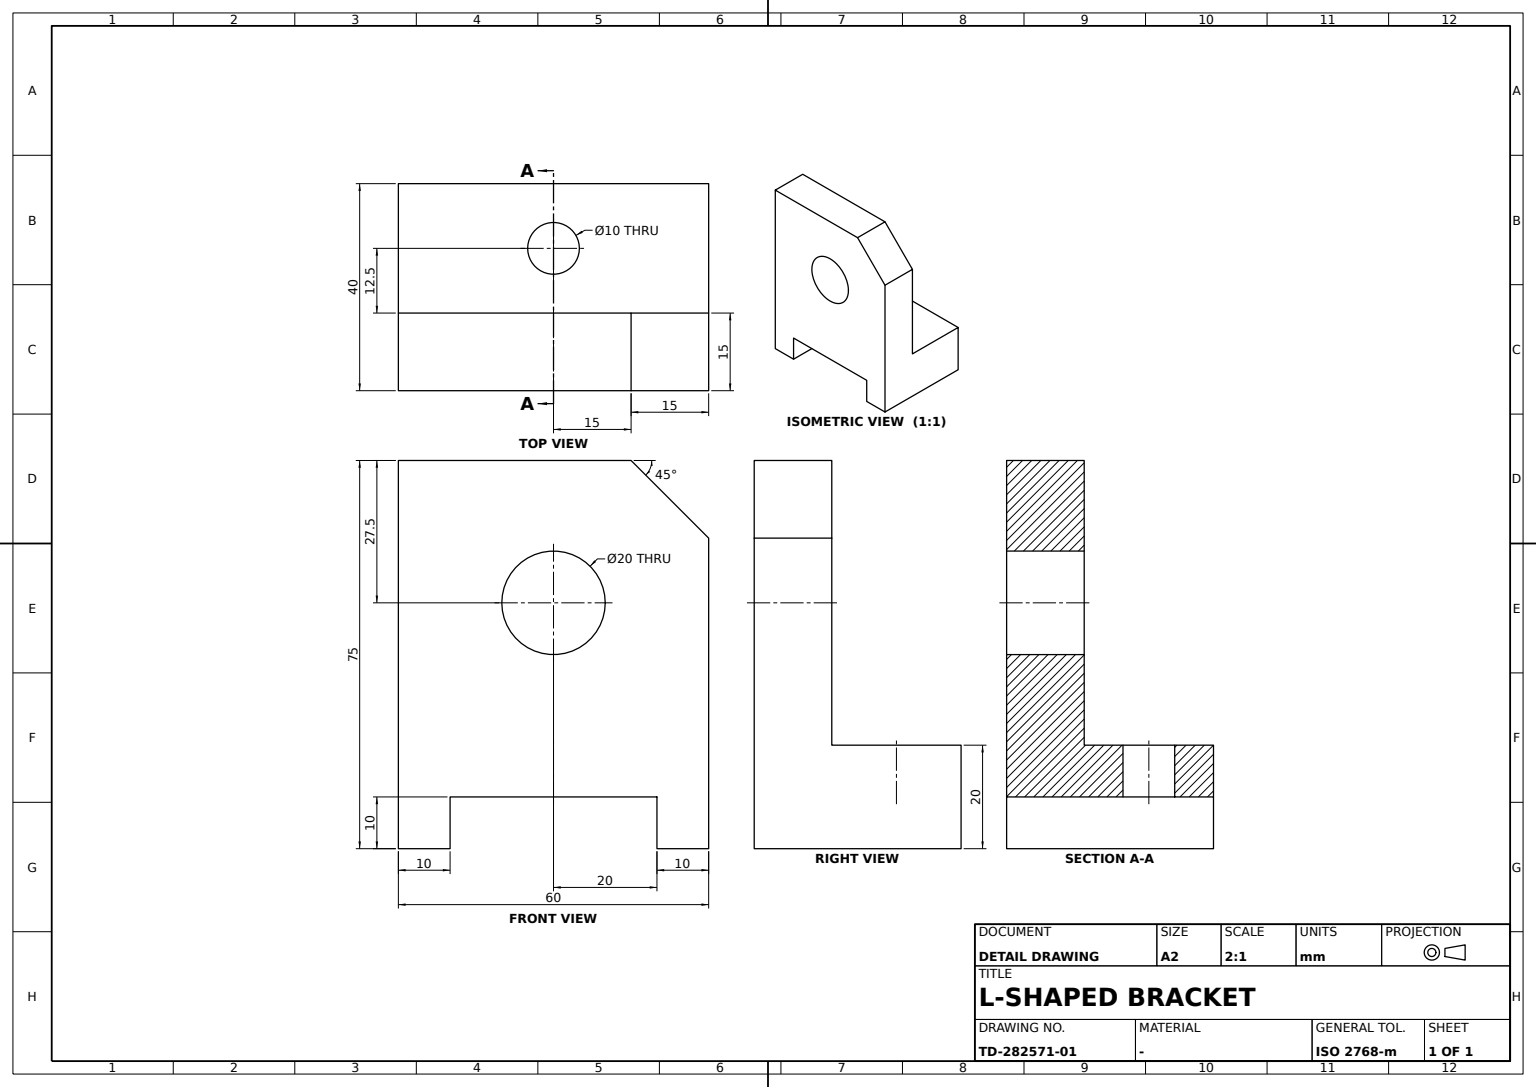
ISO-10303-21;
HEADER;
FILE_DESCRIPTION((''),'2;1');
FILE_NAME('','',(''),(''),'','','');
FILE_SCHEMA(('AUTOMOTIVE_DESIGN'));
ENDSEC;
DATA;
#1=APPLICATION_CONTEXT('');
#2=PRODUCT_CONTEXT('',#1,'mechanical');
#3=PRODUCT('','','',(#2));
#4=PRODUCT_DEFINITION_FORMATION('','',#3);
#5=PRODUCT_DEFINITION_CONTEXT('',#1,'design');
#6=PRODUCT_DEFINITION('','',#4,#5);
#7=PRODUCT_DEFINITION_SHAPE('','',#6);
#8=(LENGTH_UNIT()NAMED_UNIT(*)SI_UNIT(.MILLI.,.METRE.));
#9=(NAMED_UNIT(*)PLANE_ANGLE_UNIT()SI_UNIT($,.RADIAN.));
#10=(NAMED_UNIT(*)SI_UNIT($,.STERADIAN.)SOLID_ANGLE_UNIT());
#11=UNCERTAINTY_MEASURE_WITH_UNIT(LENGTH_MEASURE(1.E-05),#8,'distance_accuracy_value','');
#12=(GEOMETRIC_REPRESENTATION_CONTEXT(3)GLOBAL_UNCERTAINTY_ASSIGNED_CONTEXT((#11))GLOBAL_UNIT_ASSIGNED_CONTEXT((#8,#9,#10))REPRESENTATION_CONTEXT('',''));
#13=CARTESIAN_POINT('',(-20.,20.,10.));
#14=VERTEX_POINT('',#13);
#15=CARTESIAN_POINT('',(20.,20.,10.));
#16=VERTEX_POINT('',#15);
#17=CARTESIAN_POINT('',(0.,20.,10.));
#18=DIRECTION('',(1.,0.,0.));
#19=VECTOR('',#18,1000.);
#20=LINE('',#17,#19);
#21=EDGE_CURVE('',#14,#16,#20,.T.);
#22=ORIENTED_EDGE('',*,*,#21,.T.);
#23=CARTESIAN_POINT('',(20.,-20.,10.));
#24=VERTEX_POINT('',#23);
#25=CARTESIAN_POINT('',(20.,0.,10.));
#26=DIRECTION('',(0.,-1.,0.));
#27=VECTOR('',#26,1000.);
#28=LINE('',#25,#27);
#29=EDGE_CURVE('',#16,#24,#28,.T.);
#30=ORIENTED_EDGE('',*,*,#29,.T.);
#31=CARTESIAN_POINT('',(-20.,-20.,10.));
#32=VERTEX_POINT('',#31);
#33=CARTESIAN_POINT('',(0.,-20.,10.));
#34=DIRECTION('',(-1.,0.,0.));
#35=VECTOR('',#34,1000.);
#36=LINE('',#33,#35);
#37=EDGE_CURVE('',#24,#32,#36,.T.);
#38=ORIENTED_EDGE('',*,*,#37,.T.);
#39=CARTESIAN_POINT('',(-20.,0.,10.));
#40=LINE('',#39,#27);
#41=EDGE_CURVE('',#14,#32,#40,.T.);
#42=ORIENTED_EDGE('',*,*,#41,.F.);
#43=EDGE_LOOP('',(#22,#30,#38,#42));
#44=FACE_OUTER_BOUND('',#43,.T.);
#45=CARTESIAN_POINT('',(-5.,7.5,10.));
#46=VERTEX_POINT('',#45);
#47=CARTESIAN_POINT('',(5.,7.5,10.));
#48=VERTEX_POINT('',#47);
#49=CARTESIAN_POINT('',(0.,7.5,10.));
#50=DIRECTION('',(0.,0.,1.));
#51=AXIS2_PLACEMENT_3D('',#49,#50,#34);
#52=CIRCLE('',#51,5.);
#53=EDGE_CURVE('',#46,#48,#52,.T.);
#54=ORIENTED_EDGE('',*,*,#53,.T.);
#55=EDGE_CURVE('',#48,#46,#52,.T.);
#56=ORIENTED_EDGE('',*,*,#55,.T.);
#57=EDGE_LOOP('',(#54,#56));
#58=FACE_BOUND('',#57,.T.);
#59=AXIS2_PLACEMENT_3D('',#15,#50,#34);
#60=PLANE('',#59);
#61=ADVANCED_FACE('',(#44,#58),#60,.F.);
#62=ORIENTED_EDGE('',*,*,#21,.F.);
#63=CARTESIAN_POINT('',(-20.,20.,0.));
#64=VERTEX_POINT('',#63);
#65=CARTESIAN_POINT('',(-20.,20.,5.));
#66=VECTOR('',#50,1000.);
#67=LINE('',#65,#66);
#68=EDGE_CURVE('',#64,#14,#67,.T.);
#69=ORIENTED_EDGE('',*,*,#68,.F.);
#70=CARTESIAN_POINT('',(-30.,20.,0.));
#71=VERTEX_POINT('',#70);
#72=CARTESIAN_POINT('',(-25.,20.,0.));
#73=LINE('',#72,#19);
#74=EDGE_CURVE('',#71,#64,#73,.T.);
#75=ORIENTED_EDGE('',*,*,#74,.F.);
#76=CARTESIAN_POINT('',(-30.,20.,20.));
#77=VERTEX_POINT('',#76);
#78=CARTESIAN_POINT('',(-30.,20.,10.));
#79=LINE('',#78,#66);
#80=EDGE_CURVE('',#71,#77,#79,.T.);
#81=ORIENTED_EDGE('',*,*,#80,.T.);
#82=CARTESIAN_POINT('',(30.,20.,20.));
#83=VERTEX_POINT('',#82);
#84=CARTESIAN_POINT('',(0.,20.,20.));
#85=LINE('',#84,#19);
#86=EDGE_CURVE('',#77,#83,#85,.T.);
#87=ORIENTED_EDGE('',*,*,#86,.T.);
#88=CARTESIAN_POINT('',(30.,20.,0.));
#89=VERTEX_POINT('',#88);
#90=CARTESIAN_POINT('',(30.,20.,10.));
#91=LINE('',#90,#66);
#92=EDGE_CURVE('',#89,#83,#91,.T.);
#93=ORIENTED_EDGE('',*,*,#92,.F.);
#94=CARTESIAN_POINT('',(20.,20.,0.));
#95=VERTEX_POINT('',#94);
#96=CARTESIAN_POINT('',(25.,20.,0.));
#97=LINE('',#96,#19);
#98=EDGE_CURVE('',#95,#89,#97,.T.);
#99=ORIENTED_EDGE('',*,*,#98,.F.);
#100=CARTESIAN_POINT('',(20.,20.,5.));
#101=DIRECTION('',(0.,0.,-1.));
#102=VECTOR('',#101,1000.);
#103=LINE('',#100,#102);
#104=EDGE_CURVE('',#16,#95,#103,.T.);
#105=ORIENTED_EDGE('',*,*,#104,.F.);
#106=EDGE_LOOP('',(#62,#69,#75,#81,#87,#93,#99,#105));
#107=FACE_OUTER_BOUND('',#106,.T.);
#108=CARTESIAN_POINT('',(0.,20.,0.));
#109=DIRECTION('',(0.,1.,0.));
#110=AXIS2_PLACEMENT_3D('',#108,#109,#50);
#111=PLANE('',#110);
#112=ADVANCED_FACE('',(#107),#111,.T.);
#113=ORIENTED_EDGE('',*,*,#86,.F.);
#114=CARTESIAN_POINT('',(-30.,-5.,20.));
#115=VERTEX_POINT('',#114);
#116=CARTESIAN_POINT('',(-30.,7.5,20.));
#117=LINE('',#116,#27);
#118=EDGE_CURVE('',#77,#115,#117,.T.);
#119=ORIENTED_EDGE('',*,*,#118,.T.);
#120=CARTESIAN_POINT('',(30.,-5.,20.));
#121=VERTEX_POINT('',#120);
#122=CARTESIAN_POINT('',(0.,-5.,20.));
#123=LINE('',#122,#19);
#124=EDGE_CURVE('',#115,#121,#123,.T.);
#125=ORIENTED_EDGE('',*,*,#124,.T.);
#126=CARTESIAN_POINT('',(30.,7.5,20.));
#127=LINE('',#126,#27);
#128=EDGE_CURVE('',#83,#121,#127,.T.);
#129=ORIENTED_EDGE('',*,*,#128,.F.);
#130=EDGE_LOOP('',(#113,#119,#125,#129));
#131=FACE_OUTER_BOUND('',#130,.T.);
#132=CARTESIAN_POINT('',(5.,7.5,20.));
#133=VERTEX_POINT('',#132);
#134=CARTESIAN_POINT('',(-5.,7.5,20.));
#135=VERTEX_POINT('',#134);
#136=CARTESIAN_POINT('',(0.,7.5,20.));
#137=AXIS2_PLACEMENT_3D('',#136,#50,#34);
#138=CIRCLE('',#137,5.);
#139=EDGE_CURVE('',#133,#135,#138,.T.);
#140=ORIENTED_EDGE('',*,*,#139,.F.);
#141=EDGE_CURVE('',#135,#133,#138,.T.);
#142=ORIENTED_EDGE('',*,*,#141,.F.);
#143=EDGE_LOOP('',(#140,#142));
#144=FACE_BOUND('',#143,.T.);
#145=AXIS2_PLACEMENT_3D('',#84,#50,#26);
#146=PLANE('',#145);
#147=ADVANCED_FACE('',(#131,#144),#146,.T.);
#148=CARTESIAN_POINT('',(20.,-20.,0.));
#149=VERTEX_POINT('',#148);
#150=CARTESIAN_POINT('',(30.,-20.,0.));
#151=VERTEX_POINT('',#150);
#152=CARTESIAN_POINT('',(25.,-20.,0.));
#153=LINE('',#152,#19);
#154=EDGE_CURVE('',#149,#151,#153,.T.);
#155=ORIENTED_EDGE('',*,*,#154,.F.);
#156=CARTESIAN_POINT('',(20.,0.,0.));
#157=LINE('',#156,#27);
#158=EDGE_CURVE('',#95,#149,#157,.T.);
#159=ORIENTED_EDGE('',*,*,#158,.F.);
#160=ORIENTED_EDGE('',*,*,#98,.T.);
#161=CARTESIAN_POINT('',(30.,0.,0.));
#162=VECTOR('',#109,1000.);
#163=LINE('',#161,#162);
#164=EDGE_CURVE('',#151,#89,#163,.T.);
#165=ORIENTED_EDGE('',*,*,#164,.F.);
#166=EDGE_LOOP('',(#155,#159,#160,#165));
#167=FACE_OUTER_BOUND('',#166,.T.);
#168=CARTESIAN_POINT('',(0.,-20.,0.));
#169=AXIS2_PLACEMENT_3D('',#168,#101,#109);
#170=PLANE('',#169);
#171=ADVANCED_FACE('',(#167),#170,.T.);
#172=CARTESIAN_POINT('',(10.,-5.,47.5));
#173=VERTEX_POINT('',#172);
#174=CARTESIAN_POINT('',(-10.,-5.,47.5));
#175=VERTEX_POINT('',#174);
#176=CARTESIAN_POINT('',(0.,-5.,47.5));
#177=AXIS2_PLACEMENT_3D('',#176,#109,#34);
#178=CIRCLE('',#177,10.);
#179=EDGE_CURVE('',#173,#175,#178,.T.);
#180=ORIENTED_EDGE('',*,*,#179,.T.);
#181=CARTESIAN_POINT('',(-10.,-20.,47.5));
#182=VERTEX_POINT('',#181);
#183=CARTESIAN_POINT('',(-10.,-13.16,47.5));
#184=LINE('',#183,#27);
#185=EDGE_CURVE('',#175,#182,#184,.T.);
#186=ORIENTED_EDGE('',*,*,#185,.T.);
#187=CARTESIAN_POINT('',(10.,-20.,47.5));
#188=VERTEX_POINT('',#187);
#189=CARTESIAN_POINT('',(0.,-20.,47.5));
#190=AXIS2_PLACEMENT_3D('',#189,#109,#50);
#191=CIRCLE('',#190,10.);
#192=EDGE_CURVE('',#188,#182,#191,.T.);
#193=ORIENTED_EDGE('',*,*,#192,.F.);
#194=CARTESIAN_POINT('',(10.,-13.16,47.5));
#195=LINE('',#194,#27);
#196=EDGE_CURVE('',#173,#188,#195,.T.);
#197=ORIENTED_EDGE('',*,*,#196,.F.);
#198=EDGE_LOOP('',(#180,#186,#193,#197));
#199=FACE_OUTER_BOUND('',#198,.T.);
#200=CARTESIAN_POINT('',(0.,-13.16,47.5));
#201=AXIS2_PLACEMENT_3D('',#200,#26,#34);
#202=CYLINDRICAL_SURFACE('',#201,10.);
#203=ADVANCED_FACE('',(#199),#202,.F.);
#204=CARTESIAN_POINT('',(20.,-20.,5.));
#205=LINE('',#204,#66);
#206=EDGE_CURVE('',#149,#24,#205,.T.);
#207=ORIENTED_EDGE('',*,*,#206,.T.);
#208=ORIENTED_EDGE('',*,*,#29,.F.);
#209=ORIENTED_EDGE('',*,*,#104,.T.);
#210=ORIENTED_EDGE('',*,*,#158,.T.);
#211=EDGE_LOOP('',(#207,#208,#209,#210));
#212=FACE_OUTER_BOUND('',#211,.T.);
#213=AXIS2_PLACEMENT_3D('',#94,#18,#50);
#214=PLANE('',#213);
#215=ADVANCED_FACE('',(#212),#214,.F.);
#216=ORIENTED_EDGE('',*,*,#41,.T.);
#217=CARTESIAN_POINT('',(-20.,-20.,0.));
#218=VERTEX_POINT('',#217);
#219=CARTESIAN_POINT('',(-20.,-20.,5.));
#220=LINE('',#219,#66);
#221=EDGE_CURVE('',#218,#32,#220,.T.);
#222=ORIENTED_EDGE('',*,*,#221,.F.);
#223=CARTESIAN_POINT('',(-20.,0.,0.));
#224=LINE('',#223,#27);
#225=EDGE_CURVE('',#64,#218,#224,.T.);
#226=ORIENTED_EDGE('',*,*,#225,.F.);
#227=ORIENTED_EDGE('',*,*,#68,.T.);
#228=EDGE_LOOP('',(#216,#222,#226,#227));
#229=FACE_OUTER_BOUND('',#228,.T.);
#230=AXIS2_PLACEMENT_3D('',#13,#34,#101);
#231=PLANE('',#230);
#232=ADVANCED_FACE('',(#229),#231,.F.);
#233=ORIENTED_EDGE('',*,*,#206,.F.);
#234=ORIENTED_EDGE('',*,*,#154,.T.);
#235=CARTESIAN_POINT('',(30.,-20.,60.));
#236=VERTEX_POINT('',#235);
#237=CARTESIAN_POINT('',(30.,-20.,30.));
#238=LINE('',#237,#102);
#239=EDGE_CURVE('',#236,#151,#238,.T.);
#240=ORIENTED_EDGE('',*,*,#239,.F.);
#241=CARTESIAN_POINT('',(15.,-20.,75.));
#242=VERTEX_POINT('',#241);
#243=CARTESIAN_POINT('',(22.5,-20.,67.5));
#244=DIRECTION('',(0.707106781,0.,-0.707106781));
#245=VECTOR('',#244,1000.);
#246=LINE('',#243,#245);
#247=EDGE_CURVE('',#242,#236,#246,.T.);
#248=ORIENTED_EDGE('',*,*,#247,.F.);
#249=CARTESIAN_POINT('',(-30.,-20.,75.));
#250=VERTEX_POINT('',#249);
#251=CARTESIAN_POINT('',(-7.5,-20.,75.));
#252=LINE('',#251,#19);
#253=EDGE_CURVE('',#250,#242,#252,.T.);
#254=ORIENTED_EDGE('',*,*,#253,.F.);
#255=CARTESIAN_POINT('',(-30.,-20.,0.));
#256=VERTEX_POINT('',#255);
#257=CARTESIAN_POINT('',(-30.,-20.,37.5));
#258=LINE('',#257,#102);
#259=EDGE_CURVE('',#250,#256,#258,.T.);
#260=ORIENTED_EDGE('',*,*,#259,.T.);
#261=CARTESIAN_POINT('',(-25.,-20.,0.));
#262=LINE('',#261,#19);
#263=EDGE_CURVE('',#256,#218,#262,.T.);
#264=ORIENTED_EDGE('',*,*,#263,.T.);
#265=ORIENTED_EDGE('',*,*,#221,.T.);
#266=ORIENTED_EDGE('',*,*,#37,.F.);
#267=EDGE_LOOP('',(#233,#234,#240,#248,#254,#260,#264,#265,#266));
#268=FACE_OUTER_BOUND('',#267,.T.);
#269=EDGE_CURVE('',#182,#188,#191,.T.);
#270=ORIENTED_EDGE('',*,*,#269,.T.);
#271=ORIENTED_EDGE('',*,*,#192,.T.);
#272=EDGE_LOOP('',(#270,#271));
#273=FACE_BOUND('',#272,.T.);
#274=AXIS2_PLACEMENT_3D('',#168,#109,#50);
#275=PLANE('',#274);
#276=ADVANCED_FACE('',(#268,#273),#275,.F.);
#277=CARTESIAN_POINT('',(30.,-5.,60.));
#278=VERTEX_POINT('',#277);
#279=CARTESIAN_POINT('',(30.,-5.,40.));
#280=LINE('',#279,#66);
#281=EDGE_CURVE('',#121,#278,#280,.T.);
#282=ORIENTED_EDGE('',*,*,#281,.F.);
#283=ORIENTED_EDGE('',*,*,#124,.F.);
#284=CARTESIAN_POINT('',(-30.,-5.,75.));
#285=VERTEX_POINT('',#284);
#286=CARTESIAN_POINT('',(-30.,-5.,47.5));
#287=LINE('',#286,#66);
#288=EDGE_CURVE('',#115,#285,#287,.T.);
#289=ORIENTED_EDGE('',*,*,#288,.T.);
#290=CARTESIAN_POINT('',(15.,-5.,75.));
#291=VERTEX_POINT('',#290);
#292=CARTESIAN_POINT('',(-7.5,-5.,75.));
#293=LINE('',#292,#19);
#294=EDGE_CURVE('',#285,#291,#293,.T.);
#295=ORIENTED_EDGE('',*,*,#294,.T.);
#296=CARTESIAN_POINT('',(22.5,-5.,67.5));
#297=DIRECTION('',(-0.707106781,0.,0.707106781));
#298=VECTOR('',#297,1000.);
#299=LINE('',#296,#298);
#300=EDGE_CURVE('',#278,#291,#299,.T.);
#301=ORIENTED_EDGE('',*,*,#300,.F.);
#302=EDGE_LOOP('',(#282,#283,#289,#295,#301));
#303=FACE_OUTER_BOUND('',#302,.T.);
#304=EDGE_CURVE('',#175,#173,#178,.T.);
#305=ORIENTED_EDGE('',*,*,#304,.F.);
#306=ORIENTED_EDGE('',*,*,#179,.F.);
#307=EDGE_LOOP('',(#305,#306));
#308=FACE_BOUND('',#307,.T.);
#309=AXIS2_PLACEMENT_3D('',#122,#109,#50);
#310=PLANE('',#309);
#311=ADVANCED_FACE('',(#303,#308),#310,.T.);
#312=ORIENTED_EDGE('',*,*,#225,.T.);
#313=ORIENTED_EDGE('',*,*,#263,.F.);
#314=CARTESIAN_POINT('',(-30.,0.,0.));
#315=LINE('',#314,#162);
#316=EDGE_CURVE('',#256,#71,#315,.T.);
#317=ORIENTED_EDGE('',*,*,#316,.T.);
#318=ORIENTED_EDGE('',*,*,#74,.T.);
#319=EDGE_LOOP('',(#312,#313,#317,#318));
#320=FACE_OUTER_BOUND('',#319,.T.);
#321=ADVANCED_FACE('',(#320),#170,.T.);
#322=ORIENTED_EDGE('',*,*,#92,.T.);
#323=ORIENTED_EDGE('',*,*,#128,.T.);
#324=ORIENTED_EDGE('',*,*,#281,.T.);
#325=CARTESIAN_POINT('',(30.,-12.5,60.));
#326=LINE('',#325,#27);
#327=EDGE_CURVE('',#278,#236,#326,.T.);
#328=ORIENTED_EDGE('',*,*,#327,.T.);
#329=ORIENTED_EDGE('',*,*,#239,.T.);
#330=ORIENTED_EDGE('',*,*,#164,.T.);
#331=EDGE_LOOP('',(#322,#323,#324,#328,#329,#330));
#332=FACE_OUTER_BOUND('',#331,.T.);
#333=AXIS2_PLACEMENT_3D('',#161,#18,#109);
#334=PLANE('',#333);
#335=ADVANCED_FACE('',(#332),#334,.T.);
#336=CARTESIAN_POINT('',(-5.,7.5,9.34));
#337=LINE('',#336,#102);
#338=EDGE_CURVE('',#135,#46,#337,.T.);
#339=ORIENTED_EDGE('',*,*,#338,.F.);
#340=ORIENTED_EDGE('',*,*,#141,.T.);
#341=CARTESIAN_POINT('',(5.,7.5,9.34));
#342=LINE('',#341,#102);
#343=EDGE_CURVE('',#133,#48,#342,.T.);
#344=ORIENTED_EDGE('',*,*,#343,.T.);
#345=ORIENTED_EDGE('',*,*,#53,.F.);
#346=EDGE_LOOP('',(#339,#340,#344,#345));
#347=FACE_OUTER_BOUND('',#346,.T.);
#348=CARTESIAN_POINT('',(0.,7.5,9.34));
#349=AXIS2_PLACEMENT_3D('',#348,#101,#34);
#350=CYLINDRICAL_SURFACE('',#349,5.);
#351=ADVANCED_FACE('',(#347),#350,.F.);
#352=ORIENTED_EDGE('',*,*,#304,.T.);
#353=ORIENTED_EDGE('',*,*,#196,.T.);
#354=ORIENTED_EDGE('',*,*,#269,.F.);
#355=ORIENTED_EDGE('',*,*,#185,.F.);
#356=EDGE_LOOP('',(#352,#353,#354,#355));
#357=FACE_OUTER_BOUND('',#356,.T.);
#358=ADVANCED_FACE('',(#357),#202,.F.);
#359=ORIENTED_EDGE('',*,*,#288,.F.);
#360=ORIENTED_EDGE('',*,*,#118,.F.);
#361=ORIENTED_EDGE('',*,*,#80,.F.);
#362=ORIENTED_EDGE('',*,*,#316,.F.);
#363=ORIENTED_EDGE('',*,*,#259,.F.);
#364=CARTESIAN_POINT('',(-30.,-12.5,75.));
#365=LINE('',#364,#27);
#366=EDGE_CURVE('',#285,#250,#365,.T.);
#367=ORIENTED_EDGE('',*,*,#366,.F.);
#368=EDGE_LOOP('',(#359,#360,#361,#362,#363,#367));
#369=FACE_OUTER_BOUND('',#368,.T.);
#370=AXIS2_PLACEMENT_3D('',#314,#18,#109);
#371=PLANE('',#370);
#372=ADVANCED_FACE('',(#369),#371,.F.);
#373=ORIENTED_EDGE('',*,*,#300,.T.);
#374=CARTESIAN_POINT('',(15.,-12.5,75.));
#375=LINE('',#374,#27);
#376=EDGE_CURVE('',#291,#242,#375,.T.);
#377=ORIENTED_EDGE('',*,*,#376,.T.);
#378=ORIENTED_EDGE('',*,*,#247,.T.);
#379=ORIENTED_EDGE('',*,*,#327,.F.);
#380=EDGE_LOOP('',(#373,#377,#378,#379));
#381=FACE_OUTER_BOUND('',#380,.T.);
#382=CARTESIAN_POINT('',(15.,0.,75.));
#383=DIRECTION('',(0.707106781,0.,0.707106781));
#384=AXIS2_PLACEMENT_3D('',#382,#383,#26);
#385=PLANE('',#384);
#386=ADVANCED_FACE('',(#381),#385,.T.);
#387=ORIENTED_EDGE('',*,*,#253,.T.);
#388=ORIENTED_EDGE('',*,*,#376,.F.);
#389=ORIENTED_EDGE('',*,*,#294,.F.);
#390=ORIENTED_EDGE('',*,*,#366,.T.);
#391=EDGE_LOOP('',(#387,#388,#389,#390));
#392=FACE_OUTER_BOUND('',#391,.T.);
#393=CARTESIAN_POINT('',(0.,-5.,75.));
#394=AXIS2_PLACEMENT_3D('',#393,#50,#26);
#395=PLANE('',#394);
#396=ADVANCED_FACE('',(#392),#395,.T.);
#397=ORIENTED_EDGE('',*,*,#55,.F.);
#398=ORIENTED_EDGE('',*,*,#343,.F.);
#399=ORIENTED_EDGE('',*,*,#139,.T.);
#400=ORIENTED_EDGE('',*,*,#338,.T.);
#401=EDGE_LOOP('',(#397,#398,#399,#400));
#402=FACE_OUTER_BOUND('',#401,.T.);
#403=ADVANCED_FACE('',(#402),#350,.F.);
#404=CLOSED_SHELL('',(#61,#112,#147,#171,#203,#215,#232,#276,#311,#321,#335,#351,#358,#372,#386,#396,#403));
#405=MANIFOLD_SOLID_BREP('',#404);
#406=ADVANCED_BREP_SHAPE_REPRESENTATION('',(#405),#12);
#407=SHAPE_DEFINITION_REPRESENTATION(#7,#406);
ENDSEC;
END-ISO-10303-21;
